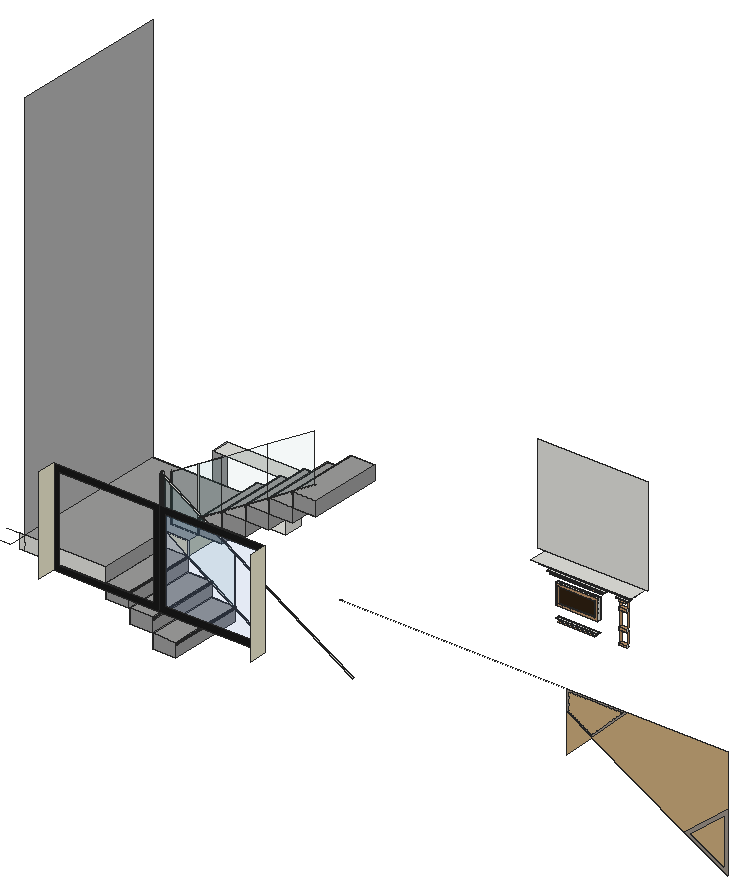
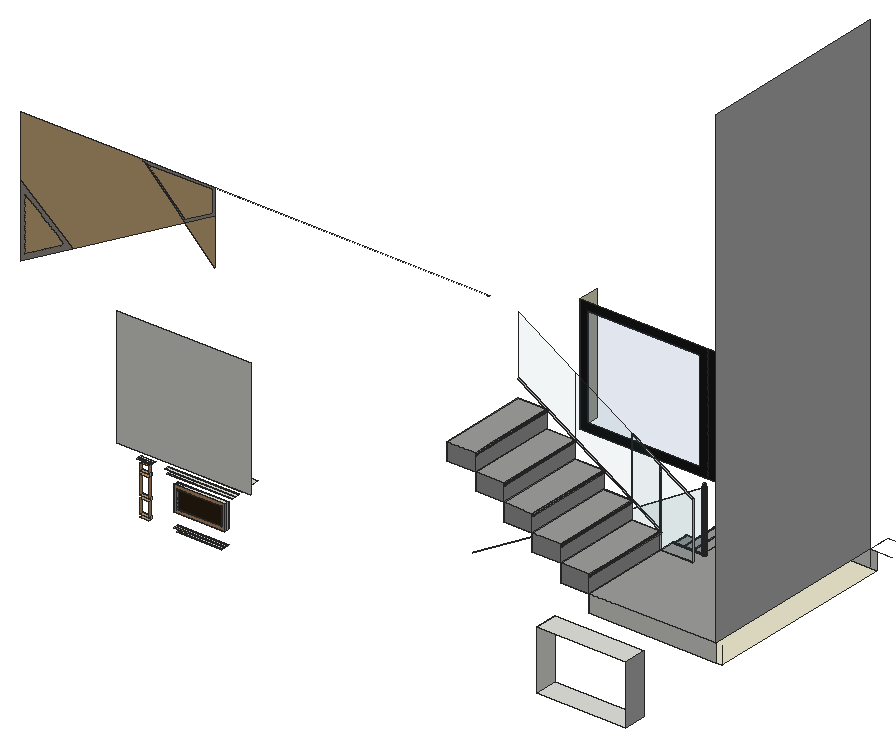
# SketchUp Ruby script. Lengths in inches.
U = 1.inch
M = Sketchup.active_model
def pt(a) = Geom::Point3d.new(a.map { |v| v * U })
def face(e, loops, mat)
  f = e.add_face(loops[0].map { |a| pt(a) })
  loops[1..].each { |l| e.add_face(l.map { |a| pt(a) }).erase! }
  f.material = f.back_material = mat if mat
  f
end
# faces: each face lists its corners as indices into pts; further lists are holes
def faces(e, pts, list, mat = nil) = list.each { |f| face(e, (f[0].is_a?(Array) ? f : [f]).map { |l| l.map { |i| pts[i] } }, mat) }
# xy, xz, yz: faces in a plane at the given z, y or x. An outline is a flat list of corners, or four numbers for a rectangle; further outlines are holes
def ring(l) = l.size == 4 ? [[l[0], l[1]], [l[2], l[1]], [l[2], l[3]], [l[0], l[3]]] : l.each_slice(2).to_a
def flat(e, list, mat, &to3) = list.each { |f| face(e, (f[0].is_a?(Array) ? f : [f]).map { |l| ring(l).map { |u, v| to3.(u, v) } }, mat) }
def xy(e, z, list, mat = nil) = flat(e, list, mat) { |x, y| [x, y, z] }
def xz(e, y, list, mat = nil) = flat(e, list, mat) { |x, z| [x, y, z] }
def yz(e, x, list, mat = nil) = flat(e, list, mat) { |y, z| [x, y, z] }
def lines(e, pts, list) = list.each { |a, b| e.add_line(pt(pts[a]), pt(pts[b])) }
# prism: a flat outline (further loops are holes) pulled along v
def prism(e, loops, v, mat = nil)
  f = face(e, loops, mat); d = Geom::Vector3d.new(v.map { |x| x * U })
  f.pushpull(f.normal.samedirection?(d) ? d.length : -d.length)
end
def box(e, o, s, mat = nil) = prism(e, [[o, [o[0] + s[0], o[1], o[2]], [o[0] + s[0], o[1] + s[1], o[2]], [o[0], o[1] + s[1], o[2]]]], [0, 0, s[2]], mat)
def at(x, y, z, deg = 0) = Geom::Transformation.translation(pt([x, y, z])) * Geom::Transformation.rotation(ORIGIN, Z_AXIS, deg.degrees)
def axes(o, x, y, z) = Geom::Transformation.new([*x, 0, *y, 0, *z, 0, *pt(o).to_a, 1])
def part(name) = M.definitions.add(name)
# library, detail: a bought-in or finely detailed component or shape, given as its bounding box
def library(name, o, s) = part(name).tap { |d| box(d.entities, o, s) }
def detail(e, o, s) = box(e.add_group.entities, o, s)
def put(e, d, t, mat = nil) = e.add_instance(d, t).tap { |i| i.material = mat if mat }
def group(e, t, mat = nil) = e.add_group.tap { |g| g.transformation = t; g.material = mat if mat }.entities
root = M.entities
M.materials.add("Drag Textured Plaster None 1500 x 1662 mm (I93S2X)").color = [206, 173, 125]
M.materials.add("Lily_Blonde").color = [237, 233, 206]
M.materials.add("Panel-Opening1").color = [191, 148, 107]
M.materials.add("Stained Mahogany").color = [48, 33, 18]
M.materials.add("Wood Wool (CH8A6D)").color = [158, 148, 138]
M.materials.add("[0136_Charcoal]").color = [25, 25, 25]
M.materials.add("[Aluminum]").color = [178, 178, 178]
M.materials.add("[Metal Silver]").color = [198, 197, 201]
M.materials.add("[Translucent Glass Blue]1").color = [97, 145, 232]
M.materials["[Translucent Glass Blue]1"].alpha = 0.15
M.materials.add("[Translucent Glass Gray]").color = [73, 161, 170]
M.materials["[Translucent Glass Gray]"].alpha = 0.06
M.materials.add("crushed-stone-asphalt-staggered-isosceles-2423-mm-architextu").color = [158, 158, 157]
c1 = part("Stair tread")
xy(c1.entities,0,[[0,0,11.5,36]])
xy(c1.entities,7,[[0,0,11.5,36]])
xz(c1.entities,0,[[0,0,11.5,7],[11.5,6,11.63,6.02,11.75,6.07,11.85,6.15,11.93,6.25,11.98,6.37,12,6.5,11.98,6.63,11.93,6.75,11.85,6.85,11.75,6.93,11.63,6.98,11.5,7]])
xz(c1.entities,36,[[0,0,11.5,7],[11.5,6,11.5,7,11.63,6.98,11.75,6.93,11.85,6.85,11.93,6.75,11.98,6.63,12,6.5,11.98,6.37,11.93,6.25,11.85,6.15,11.75,6.07,11.63,6.02]])
yz(c1.entities,0,[[0,0,36,7]])
yz(c1.entities,11.5,[[0,0,36,6],[0,6,10.3125,7],[10.3125,6,36,7]])
p = [[11.5,36,6],[11.63,36,6.02],[11.63,0,6.02],[11.5,0,6],[11.5,10.3125,6],[11.75,36,6.07],
  [11.75,0,6.07],[11.85,36,6.15],[11.85,0,6.15],[11.93,36,6.25],[11.93,0,6.25],[11.98,36,6.37],
  [11.98,0,6.37],[12,36,6.5],[12,0,6.5],[11.98,36,6.63],[11.98,0,6.63],[11.93,36,6.75],
  [11.93,0,6.75],[11.85,36,6.85],[11.85,0,6.85],[11.75,36,6.93],[11.63,36,6.98],[11.63,0,6.98],
  [11.75,0,6.93],[11.5,36,7],[11.5,10.3125,7],[11.5,0,7]]
faces(c1.entities,p,[[0,1,2,3,4],[1,5,6,2],[5,7,8,6],[7,9,10,8],[9,11,12,10],[11,13,14,12],[13,15,16,14],[15,17,18,16],
  [17,19,20,18],[21,22,23,24],[19,21,24,20],[25,26,27,23,22]])
xy(root,77,[[24,125.1875,60,134.1875]])
xy(root,82.37,[[189.57,130.4,207.91,131.15]])
xy(root,82.37,[[189.57,129.66,207.91,130.4],[219.32,130.03,223.07,131.53],[189.57,131.15,207.91,131.53]],"Panel-Opening1")
xy(root,83.52,[[188.45,130.03,209.03,131.15]])
xy(root,83.52,[[188.45,129.66,209.03,130.03],[219.32,130.03,223.07,131.53],[188.45,131.15,209.03,131.53]],"Panel-Opening1")
xy(root,89.26,[[188.45,130.03,209.03,131.15]])
xy(root,89.26,[[188.45,129.66,209.03,130.03],[219.32,130.03,223.07,131.53],[188.45,131.15,209.03,131.53]],"Panel-Opening1")
xy(root,90.41,[[189.57,130.4,207.91,131.15]])
xy(root,90.41,[[189.57,129.66,207.91,130.4],[219.32,130.03,223.07,131.53],[189.57,131.15,207.91,131.53]],"Panel-Opening1")
xy(root,94.02,[[59.59,64.6875,60.42,65.1875]])
xy(root,94.02,[[6.42,29.1875,6.42,107.1875,60.42,107.1875,60.42,65.1875,48.42,65.1875,48.42,29.1875]],"Lily_Blonde")
xy(root,98.07,[[189.57,130.4,207.91,131.15]])
xy(root,98.07,[[189.57,129.66,207.91,130.4],[219.32,130.03,223.07,131.53],[189.57,131.15,207.91,131.53]],"Panel-Opening1")
xy(root,99.22,[[188.45,130.03,209.03,131.15]])
xy(root,99.22,[[188.45,129.66,209.03,130.03],[219.32,130.03,223.07,131.53],[188.45,131.15,209.03,131.53]],"Panel-Opening1")
xy(root,101,[[24,125.1875,60,134.1875]])
xy(root,101.02,[[48.42,64.6875,60.42,65.1875],[47.23,70.6875,60.42,71.125]])
xy(root,101.02,[[[9,29.1875,48.42,29.1875,48.42,65.1875,60.42,65.1875,60.42,70.6875,47.23,70.6875,47.23,71.125,60.42,71.125,60.42,107.1875,9,107.1875],[47.5,64.13,47.3,64.16,47.12,64.23,46.96,64.35,46.85,64.51,46.77,64.6875,46.75,64.88,46.77,65.07,46.85,65.26,46.96,65.41,47.12,65.53,47.3,65.6,47.5,65.63,47.6875,65.6,47.87,65.53,48.03,65.41,48.14,65.26,48.22,65.07,48.25,64.88,48.22,64.6875,48.14,64.51,48.03,64.35,47.87,64.23,47.6875,64.16]]],"crushed-stone-asphalt-staggered-isosceles-2423-mm-architextu")
xy(root,102.09,[[185.64,130.03,211.84,131.15]])
xy(root,102.09,[[185.64,129.66,211.84,130.03],[219.32,129.66,223.07,130.59],[219.32,130.59,223.07,131.53],[185.64,131.15,211.84,131.53]],"Panel-Opening1")
xy(root,103.24,[[184.52,129.66,212.96,131.15],[218.2,129.66,224.1875,130.4],[218.2,130.4,224.1875,131.15]])
xy(root,103.24,[[184.52,131.15,212.96,131.53],[218.2,131.15,224.1875,131.53]],"Panel-Opening1")
xy(root,103.24,[[184.52,129.28,212.96,129.66],[218.2,129.28,224.1875,129.66]],"Stained Mahogany")
xy(root,105.92,[[181.9,129.28,215.58,131.15],[215.58,129.28,226.81,131.15]])
xy(root,105.92,[[181.9,127.41,226.81,129.28]],"Stained Mahogany")
xy(root,107.84,[[180.03,127.41,228.68,131.15]],"Stained Mahogany")
xy(root,108,[[180.03,125.1875,229,134.1875]])
xy(root,125.58,[[[47.5,64.13,47.6875,64.16,47.87,64.23,48.03,64.35,48.14,64.51,48.22,64.6875,48.25,64.88,48.22,65.07,48.14,65.26,48.03,65.41,47.87,65.53,47.6875,65.6,47.5,65.63,47.3,65.6,47.12,65.53,46.96,65.41,46.85,65.26,46.77,65.07,46.75,64.88,46.77,64.6875,46.85,64.51,46.96,64.35,47.12,64.23,47.3,64.16],[47.53,64.43,47.11,64.71,47.15,65.21,47.6,65.43,48.01,65.15,47.98,64.65]]],"[Metal Silver]")
xy(root,126.08,[[47.6,64.46,47.66,64.46,47.78,64.49,47.89,64.55,47.98,64.63,48.04,64.73,48.08,64.85,48.08,64.97,48.06,65.09,48,65.19,47.92,65.28,47.8125,65.35,47.7,65.38,47.66,65.39,48.01,65.15,47.98,64.65],[47.36,65.31,47.47,65.37,47.46,65.36]])
xy(root,126.08,[[47.53,64.43,47.6,64.46,47.54,64.47,47.42,64.5,47.32,64.57],[47.32,64.57,47.24,64.66,47.18,64.76,47.16,64.88,47.16,65,47.2,65.12,47.26,65.22,47.35,65.31,47.15,65.21,47.11,64.71],[47.47,65.37,47.58,65.39,47.66,65.39,47.6,65.43]],"[Metal Silver]")
xy(root,126.77,[[47.6,64.46,47.98,64.65,48.01,65.15,47.66,65.39,47.58,65.39,47.47,65.37,47.36,65.31,47.35,65.31,47.26,65.22,47.2,65.12,47.16,65,47.16,64.88,47.18,64.76,47.24,64.66,47.32,64.57,47.42,64.5,47.54,64.47]],"[Metal Silver]")
xz(root,20.1875,[[[30,97.03,81.85,144],[32.83,99.86,79.02,141.17]],[[81.85,97.03,133.71,144],[85.05,100.23,130.51,140.8]]],"[0136_Charcoal]")
xz(root,20.1875,[[85.05,100.23,130.51,140.8]],"[Translucent Glass Blue]1")
xz(root,20.75,[[358.09,81.75,358.09,103.7,342.0625,90.71],[338.67,90.42,360,107.71,360,132.8125,310.86,132.8125,293.44,115.74],[281.1875,103.73,293.44,115.74,281.1875,122.59],[293.3,116.8,308.75,131.95,282.05,131.95,282.05,123.1]],"Drag Textured Plaster None 1500 x 1662 mm (I93S2X)")
xz(root,20.75,[[[360,78.49,360,107.71,338.67,90.42],[358.09,81.75,342.0625,90.71,358.09,103.7]],[[293.44,115.74,310.86,132.8125,169.71,132.8125,169.71,132.6875,281.1875,132.6875,281.1875,122.59],[293.3,116.8,282.05,123.1,282.05,131.95,308.75,131.95]]],"Wood Wool (CH8A6D)")
xz(root,29.1875,[[6.42,94.02,9,101.02],[9,94.02,48.42,101.02]])
xz(root,64.6875,[[83.48,79.25,83.48,103.25,48.42,125.02,48.42,101.02,60.42,101.02,60.42,94.02,59.59,94.02,71.98,86.25]],"[Translucent Glass Gray]")
xz(root,65.1875,[[48.42,94.02,59.59,94.02,48.42,101.02]])
xz(root,65.1875,[[59.59,94.02,60.42,94.02,60.42,101.02,48.42,101.02]],"Lily_Blonde")
xz(root,65.1875,[[83.48,79.25,71.98,86.25,59.59,94.02,60.42,94.02,60.42,101.02,48.42,101.02,48.42,125.02,83.48,103.25]],"[Translucent Glass Gray]")
xz(root,65.39,[[47.58,126.08,47.66,126.77]],"[Metal Silver]")
xz(root,70.6875,[[60.42,108.1,71.92,115.09,71.92,139.02,60.42,132.02],[71.92,115.09,94.82,129,94.82,153,71.92,139.02],[94.82,129,117.92,143.04,117.92,167.02,94.82,153]],"[Translucent Glass Gray]")
xz(root,71.125,[[47.23,101.02,60.42,101.02,60.42,132.02,47.23,123.99]],"[Translucent Glass Gray]")
xz(root,71.1875,[[60.42,108.1,60.42,132.02,71.92,139.02,71.92,115.09]],"[Translucent Glass Gray]")
xz(root,107.1875,[[9,94.02,60.42,101.02]])
xz(root,129.66,[[[188.45,89.26,209.03,99.22],[189.57,90.41,207.91,98.07]]],"Panel-Opening1")
xz(root,130.03,[[219.32,82.37,223.07,83.52],[219.32,89.26,223.07,90.41],[219.32,98.07,223.07,99.22]],"Panel-Opening1")
xz(root,130.4,[[189.57,90.41,207.91,98.07]],"Stained Mahogany")
xz(root,131.15,[[189.57,90.41,207.91,98.07]],"Stained Mahogany")
xz(root,131.53,[[[188.45,89.26,209.03,99.22],[189.57,90.41,207.91,98.07]]],"Panel-Opening1")
xz(root,134.1875,[[176,108,230,156]])
yz(root,9,[[29.1875,101.02,107.1875,293]],"[Aluminum]")
yz(root,24,[[125.1875,77,134.1875,101]],"[Aluminum]")
yz(root,30,[[11.4375,97.03,20.1875,144]],"Lily_Blonde")
yz(root,47.16,[[64.88,126.08,65,126.77]],"[Metal Silver]")
yz(root,47.23,[[70.6875,101.02,71.125,123.99]])
yz(root,48.42,[[64.6875,101.02,65.1875,125.02]])
yz(root,48.42,[[29.1875,94.02,65.1875,101.02]],"crushed-stone-asphalt-staggered-isosceles-2423-mm-architextu")
yz(root,60,[[125.1875,77,134.1875,101]])
yz(root,60.42,[[64.6875,94.02,65.1875,101.02],[70.6875,101.02,71.125,108.1],[70.6875,108.1,71.125,132.02],[71.125,108.1,71.1875,132.02]])
yz(root,60.42,[[65.1875,94.02,107.1875,101.02]],"Lily_Blonde")
yz(root,133.71,[[11.4375,97.03,20.1875,144]],"Lily_Blonde")
yz(root,188.45,[[130.03,89.26,131.15,99.22]])
yz(root,188.45,[[129.66,89.26,130.03,99.22],[131.15,89.26,131.53,99.22]],"Panel-Opening1")
yz(root,189.57,[[130.4,90.41,131.15,98.07]])
yz(root,189.57,[[129.66,90.41,130.4,98.07],[131.15,90.41,131.53,98.07]],"Panel-Opening1")
yz(root,207.91,[[130.4,90.41,131.15,98.07]])
yz(root,207.91,[[129.66,90.41,130.4,98.07],[131.15,90.41,131.53,98.07]],"Panel-Opening1")
yz(root,209.03,[[130.03,89.26,131.15,99.22]])
yz(root,209.03,[[129.66,89.26,130.03,99.22],[131.15,89.26,131.53,99.22]],"Panel-Opening1")
yz(root,219.32,[[130.03,82.37,130.59,83.52],[130.03,89.26,130.59,90.41],[130.03,98.07,130.59,99.22],[130.59,98.07,131.15,99.22]])
yz(root,219.32,[[130.59,83.52,131.53,89.26],[130.59,90.41,131.53,98.07],[130.59,99.22,131.53,102.09]],"Panel-Opening1")
yz(root,223.07,[[130.03,82.37,130.59,83.52],[130.03,89.26,130.59,90.41],[130.03,98.07,130.59,99.22],[130.59,98.07,131.15,99.22]])
yz(root,223.07,[[130.59,83.52,131.53,89.26],[130.59,90.41,131.53,98.07],[130.59,99.22,131.53,102.09]],"Panel-Opening1")
p = [[141.27,65.1875,68.96],[118.07,65.1875,82.64],[118.07,64.6875,82.64],[141.27,64.6875,68.96],[83.48,65.1875,79.25],[94.98,65.1875,72.25],
  [94.98,64.6875,72.25],[83.48,64.6875,79.25],[71.98,65.1875,86.25],[71.98,64.6875,86.25],[83.48,65.1875,103.25],[83.48,64.6875,103.25],
  [59.59,65.1875,94.02],[59.59,64.6875,94.02],[47.3,64.16,101.02],[47.5,64.13,101.02],[47.5,64.13,125.58],[47.3,64.16,125.58],
  [47.6875,64.16,101.02],[47.6875,64.16,125.58],[46.96,64.35,101.02],[47.12,64.23,101.02],[47.12,64.23,125.58],[46.96,64.35,125.58],
  [47.87,64.23,101.02],[47.87,64.23,125.58],[48.03,64.35,101.02],[48.03,64.35,125.58],[46.85,64.51,101.02],[46.85,64.51,125.58],
  [48.14,64.51,101.02],[48.14,64.51,125.58],[46.77,64.6875,101.02],[46.77,64.6875,125.58],[48.22,64.6875,101.02],[48.22,64.6875,125.58],
  [46.75,64.88,101.02],[46.75,64.88,125.58],[48.25,64.88,101.02],[48.25,64.88,125.58],[46.77,65.07,101.02],[46.77,65.07,125.58],
  [48.22,65.07,101.02],[48.22,65.07,125.58],[46.85,65.26,101.02],[46.85,65.26,125.58],[48.14,65.26,101.02],[48.14,65.26,125.58],
  [46.96,65.41,101.02],[46.96,65.41,125.58],[48.03,65.41,101.02],[48.03,65.41,125.58],[47.12,65.53,101.02],[47.12,65.53,125.58],
  [47.87,65.53,101.02],[47.87,65.53,125.58],[47.3,65.6,101.02],[47.3,65.6,125.58],[47.6875,65.6,101.02],[47.6875,65.6,125.58],
  [47.5,65.63,101.02],[47.5,65.63,125.58],[48.42,65.1875,125.02],[48.42,64.6875,125.02],[60.42,71.1875,108.1],[71.92,71.1875,115.09],
  [71.92,70.6875,115.09],[60.42,70.6875,108.1],[60.42,71.125,108.1],[94.82,71.1875,129],[94.82,70.6875,129],[60.42,70.6875,132.02],
  [47.23,70.6875,123.99],[47.23,71.125,123.99],[60.42,71.125,132.02],[47.53,64.43,126.08],[47.32,64.57,126.08],[47.11,64.71,126.08],
  [47.11,64.71,125.58],[47.53,64.43,125.58],[47.98,64.65,126.08],[47.6,64.46,126.08],[47.98,64.65,125.58],[48.01,65.15,126.08],
  [48.01,65.15,125.58],[47.15,65.21,126.08],[47.15,65.21,125.58],[47.6,65.43,126.08],[47.66,65.39,126.08],[47.6,65.43,125.58],
  [47.35,65.31,126.08],[47.35,65.31,126.77],[47.36,65.31,126.77],[47.36,65.31,126.08],[47.47,65.37,126.08],[47.42,64.5,126.08],
  [47.42,64.5,126.77],[47.32,64.57,126.77],[47.54,64.47,126.08],[47.54,64.47,126.77],[47.6,64.46,126.77],[47.98,64.65,126.77],
  [47.24,64.66,126.08],[47.24,64.66,126.77],[48.01,65.15,126.77],[47.18,64.76,126.08],[47.18,64.76,126.77],[47.16,64.88,126.08],
  [47.16,64.88,126.77],[47.2,65.12,126.08],[47.16,65,126.08],[47.16,65,126.77],[47.2,65.12,126.77],[47.26,65.22,126.08],
  [47.26,65.22,126.77],[47.66,65.39,126.77],[47.47,65.37,126.77],[47.58,65.39,126.08],[47.58,65.39,126.77],[117.92,71.1875,143.04],
  [117.92,70.6875,143.04],[71.92,71.1875,139.02],[60.42,71.1875,132.02],[71.92,70.6875,139.02],[6.42,107.1875,94.02],[6.42,107.1875,101.02],
  [9,29.1875,101.02],[9,20.1875,101.02],[6.42,29.1875,101.02],[0,29.1875,101.02],[0,20.1875,101.02],[60.17,71.1875,107.95],
  [71.92,71.1875,115.02],[60.42,71.1875,108.02],[60.42,71.1875,101.02],[47.23,71.1875,101.02],[47.23,71.1875,125.02]]
faces(root,p,[[0,1,2,3],[4,5,6,7],[8,4,7,9],[1,10,11,2],[12,8,9,13],[10,62,63,11],[64,65,66,67,68],[65,69,70,66],
  [71,72,73,74],[69,119,120,70],[121,122,74,71,123]])
faces(root,p,[[14,15,16,17],[15,18,19,16],[20,21,22,23],[21,14,17,22],[18,24,25,19],[24,26,27,25],[28,20,23,29],[26,30,31,27],
  [32,28,29,33],[30,34,35,31],[36,32,33,37],[34,38,39,35],[40,36,37,41],[38,42,43,39],[44,40,41,45],[42,46,47,43],
  [48,44,45,49],[46,50,51,47],[52,48,49,53],[50,54,55,51],[56,52,53,57],[54,58,59,55],[60,56,57,61],[58,60,61,59],
  [75,76,77,78,79],[80,81,75,79,82],[83,80,82,84],[77,85,86,78],[87,88,83,84,89],[85,90,91,92,93,94,87,89,86],[76,95,96,97],[95,98,99,96],
  [98,81,100,99],[81,80,101,100],[102,76,97,103],[80,83,104,101],[105,102,103,106],[107,105,106,108],[109,110,111,112],[113,109,112,114],
  [83,88,115,104],[90,113,114,91],[94,93,92,116],[117,94,116,118]],"[Metal Silver]")
lines(root,p,[[124,125],[126,127],[128,129],[130,127],[131,64],[132,65],[133,64],[134,135],[135,136]])
put(root,c1,at(71.55,29.1875,73),"crushed-stone-asphalt-staggered-isosceles-2423-mm-architextu")
put(root,c1,at(60.05,29.1875,80),"crushed-stone-asphalt-staggered-isosceles-2423-mm-architextu")
put(root,c1,at(48.42,29.1875,87.02),"crushed-stone-asphalt-staggered-isosceles-2423-mm-architextu")
put(root,c1,at(71.92,107.1875,101.02,-180),"crushed-stone-asphalt-staggered-isosceles-2423-mm-architextu")
put(root,c1,at(83.42,107.1875,108.02,-180),"crushed-stone-asphalt-staggered-isosceles-2423-mm-architextu")
put(root,c1,at(94.92,107.1875,115.02,-180),"crushed-stone-asphalt-staggered-isosceles-2423-mm-architextu")
put(root,c1,at(106.42,107.1875,122.02,-180),"crushed-stone-asphalt-staggered-isosceles-2423-mm-architextu")
put(root,c1,at(117.92,107.1875,129.02,-180),"crushed-stone-asphalt-staggered-isosceles-2423-mm-architextu")
